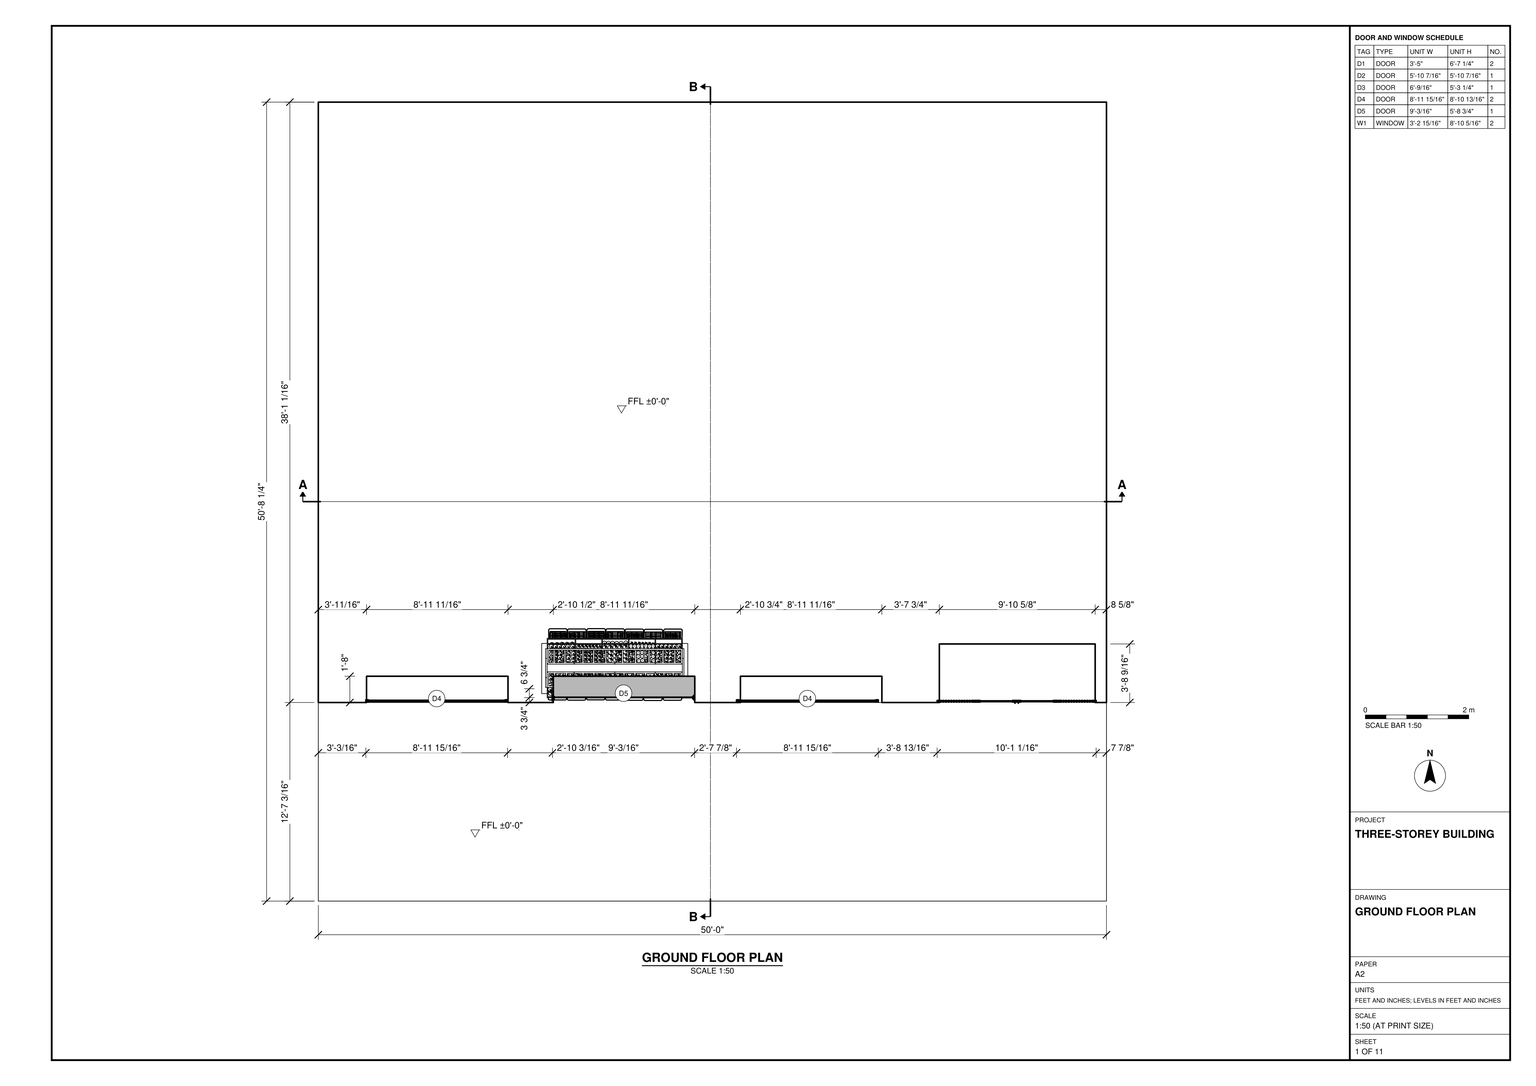
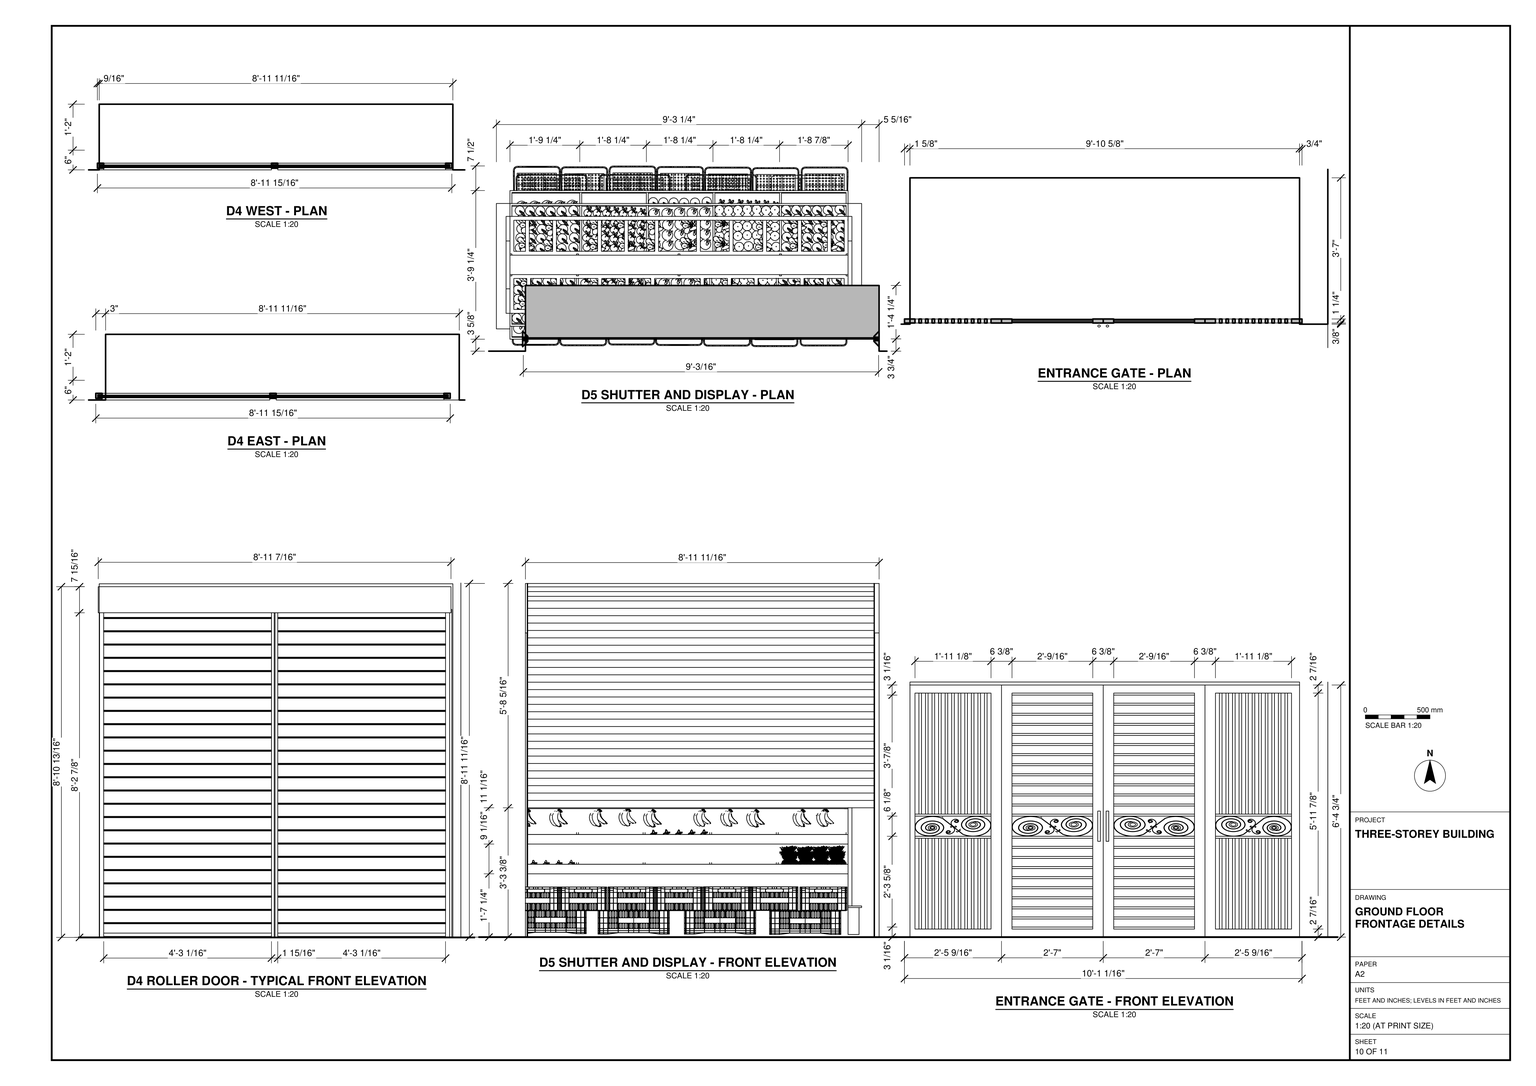
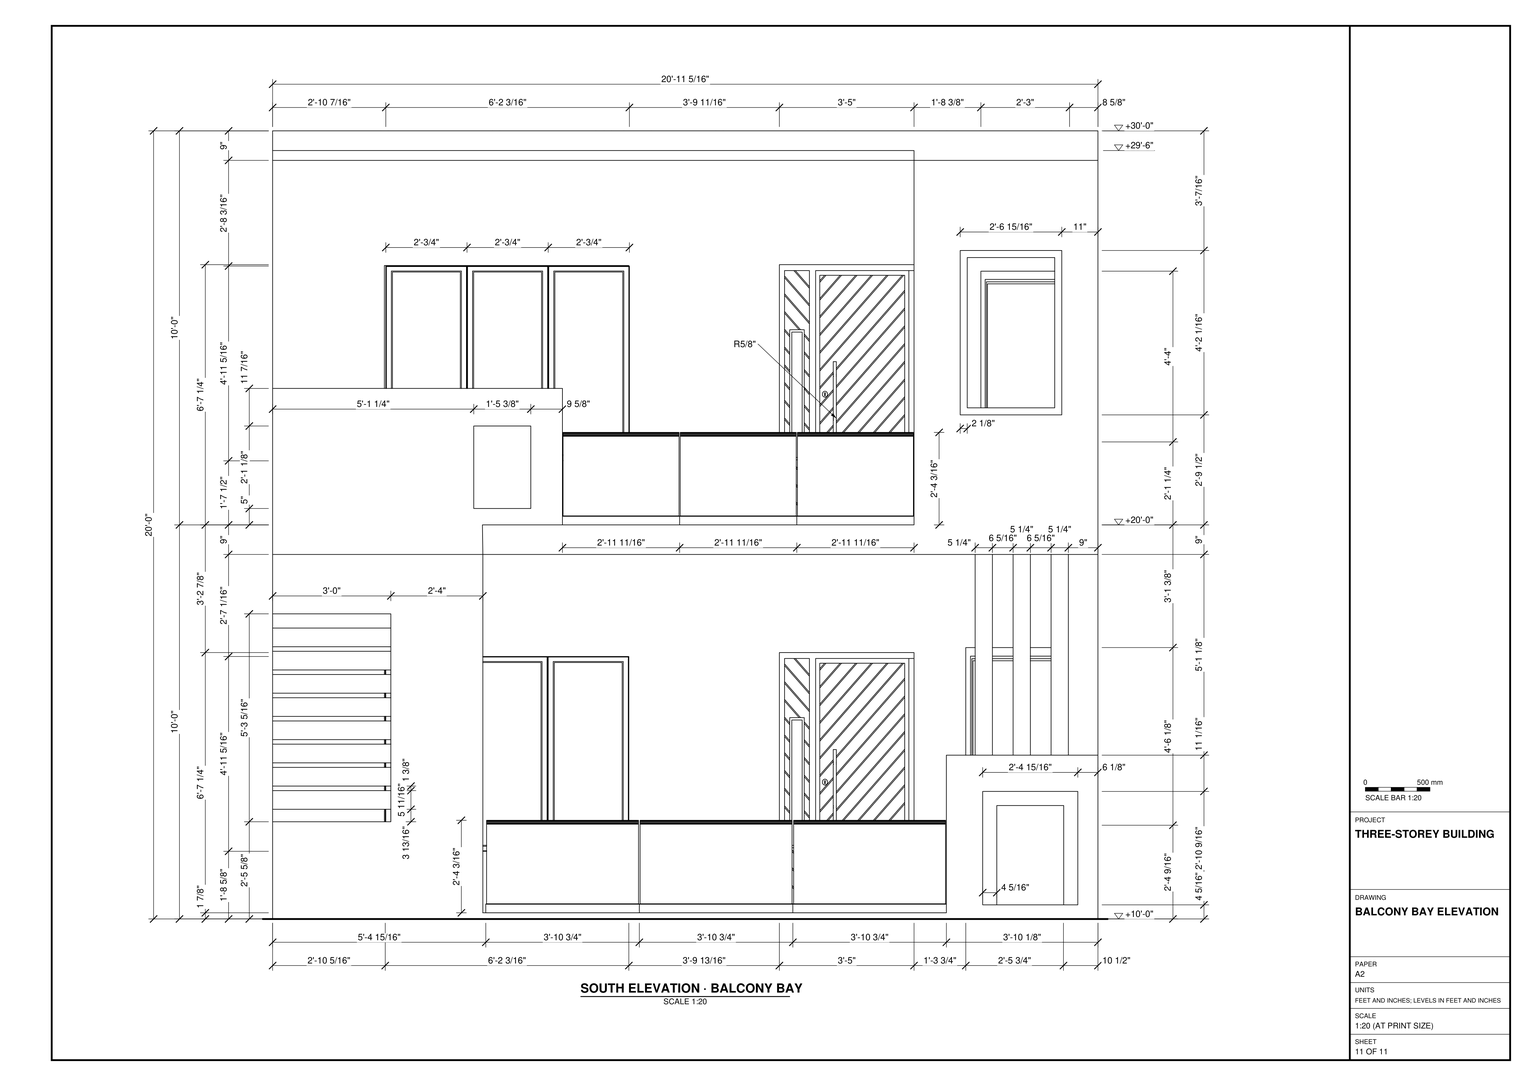
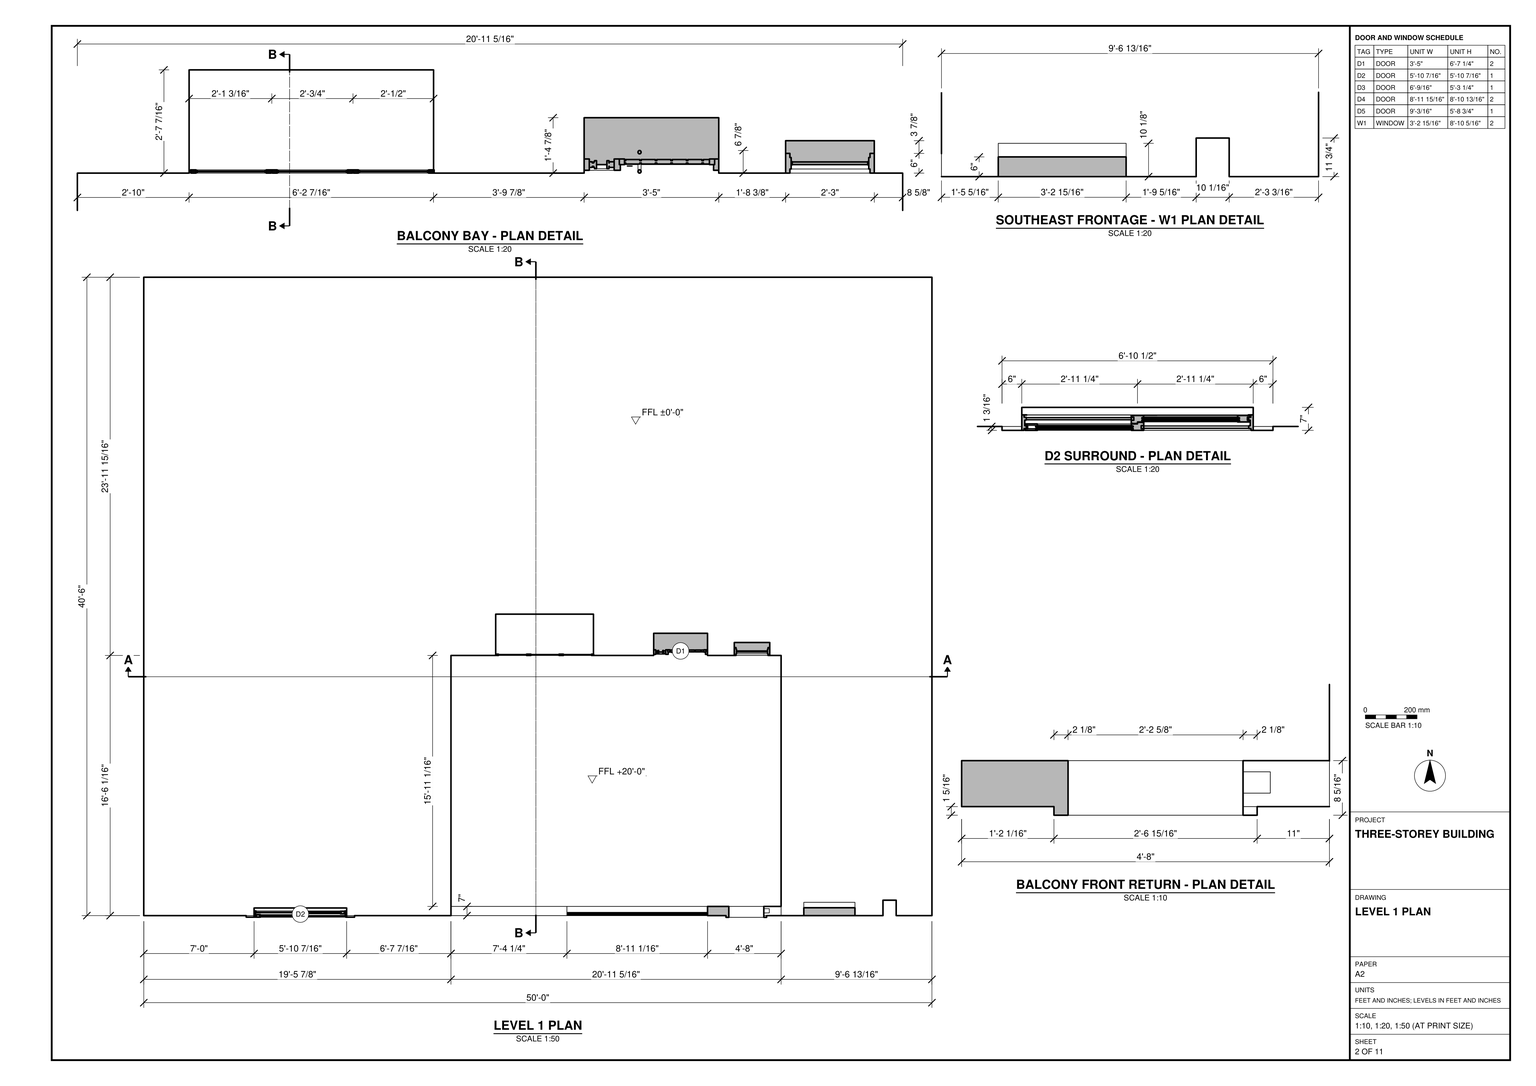
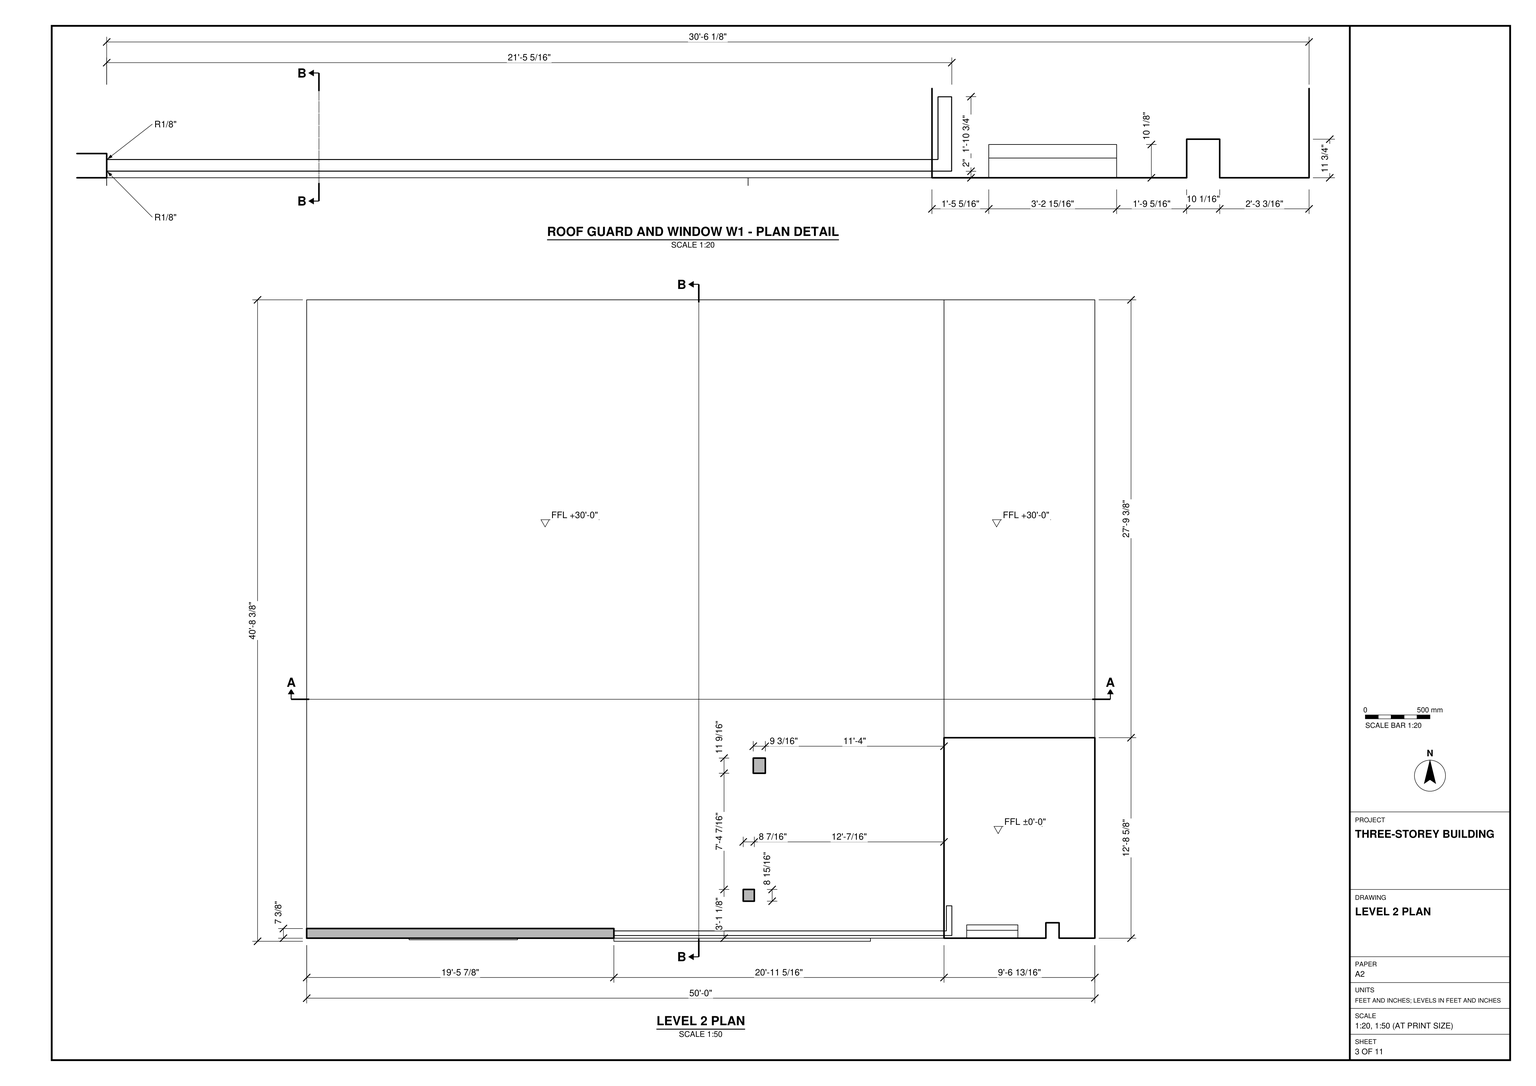
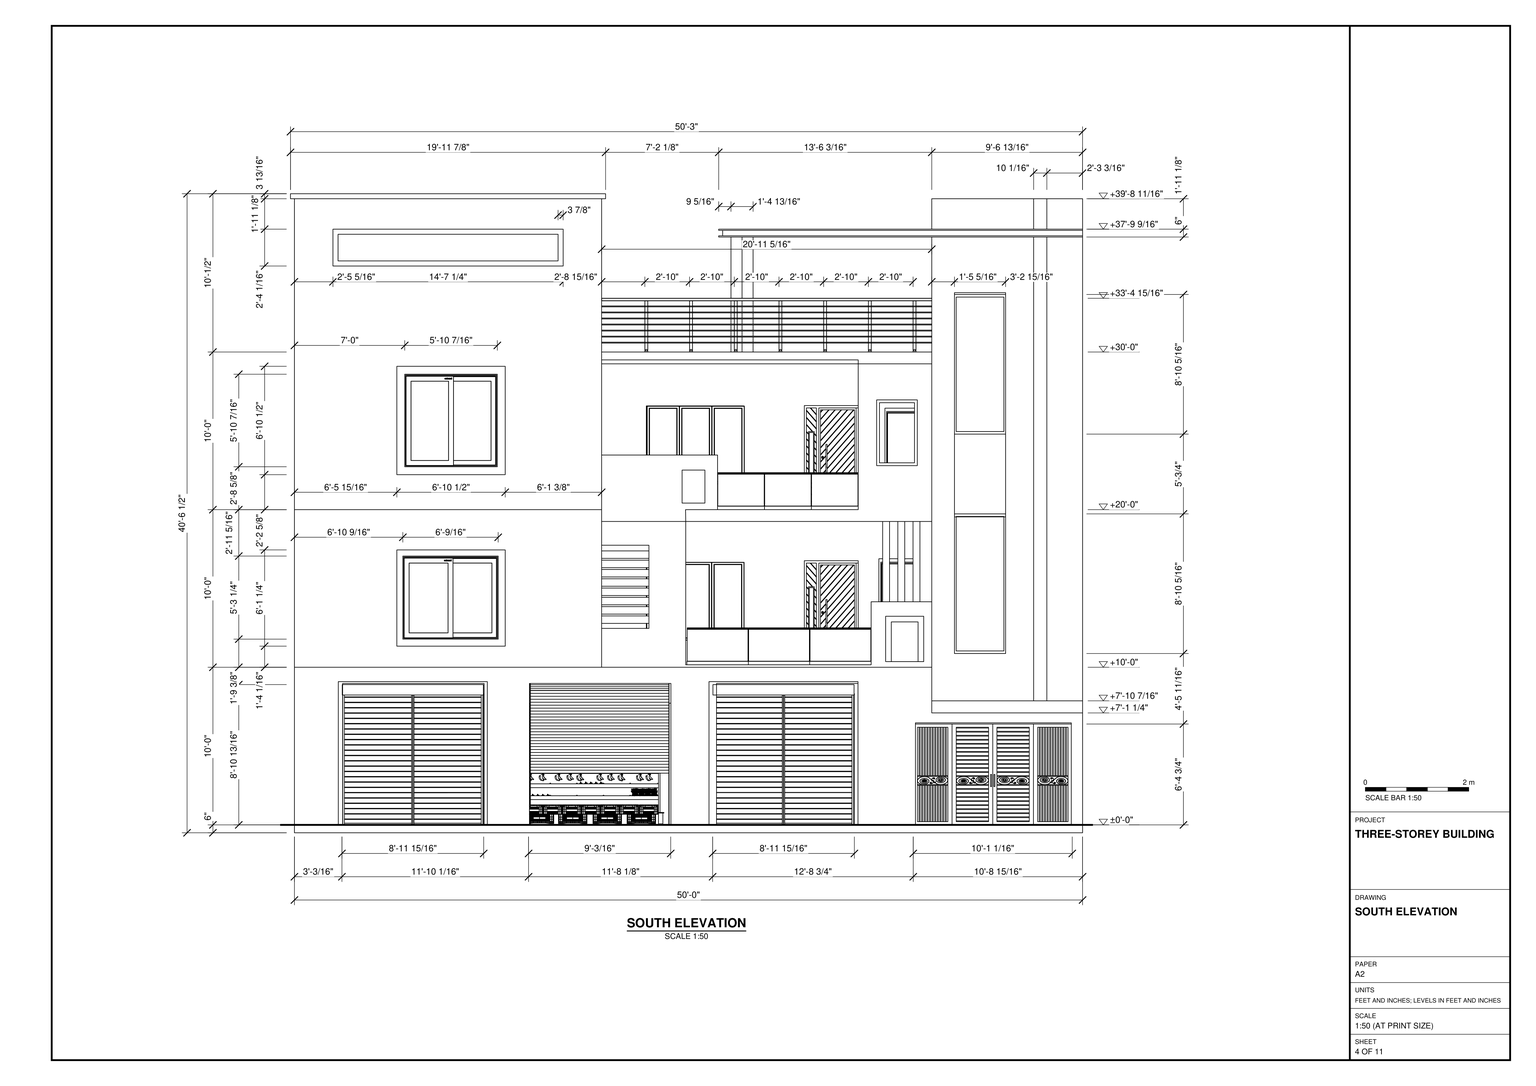
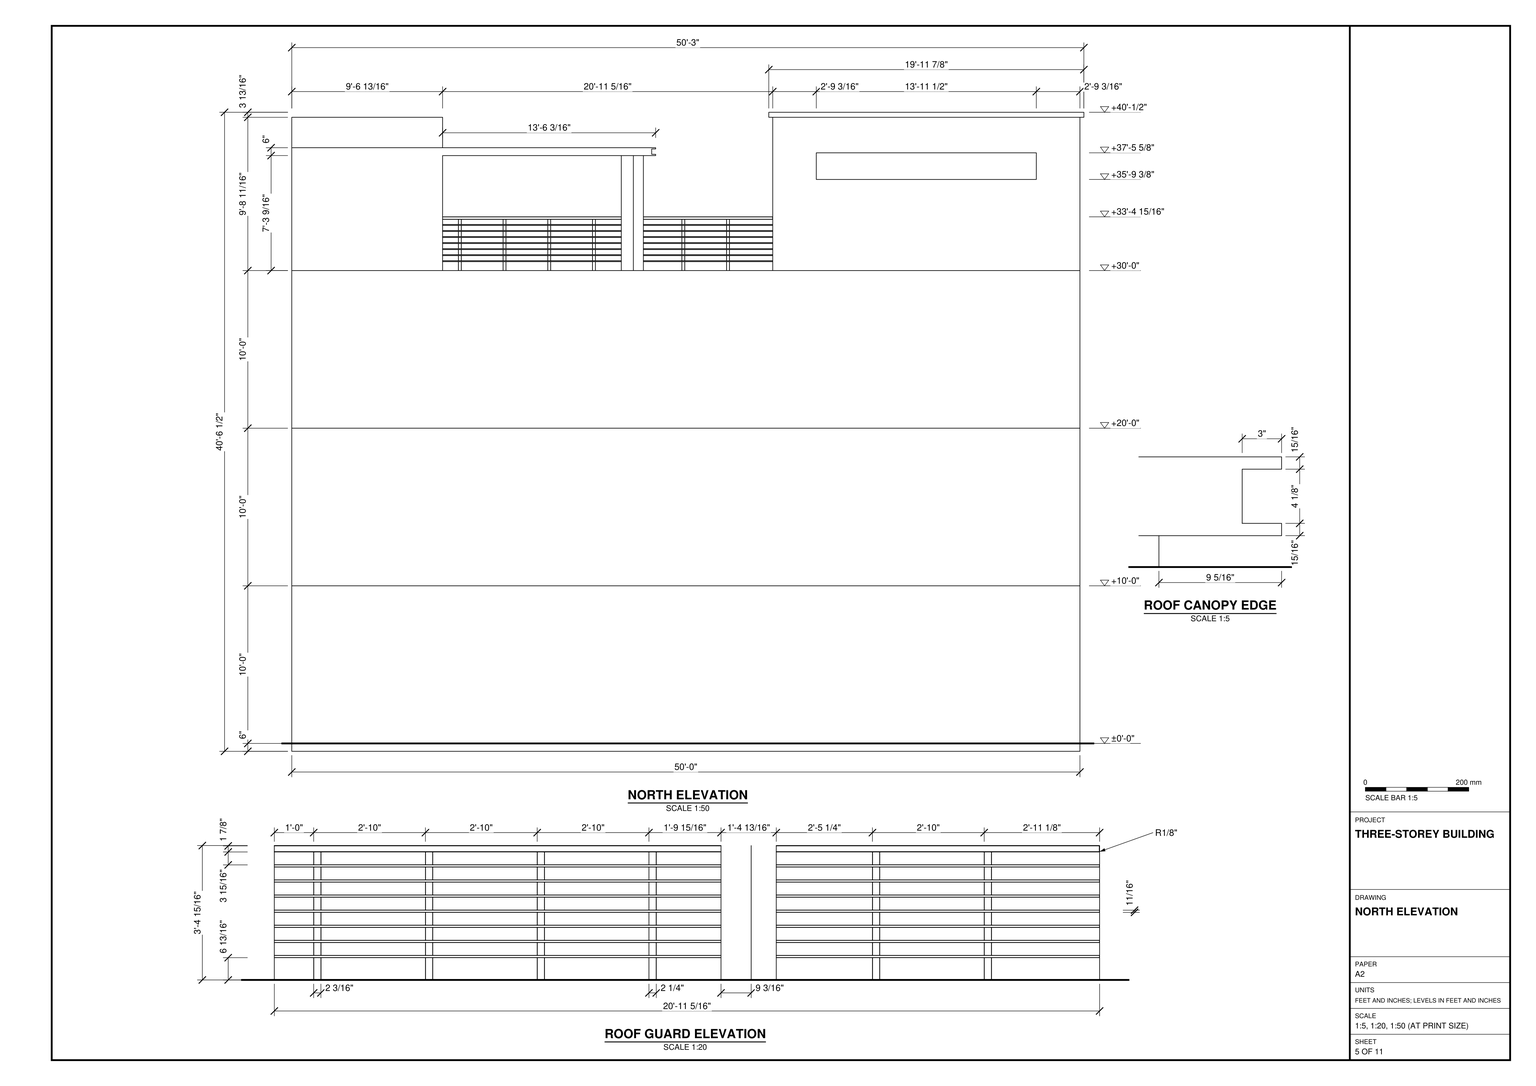
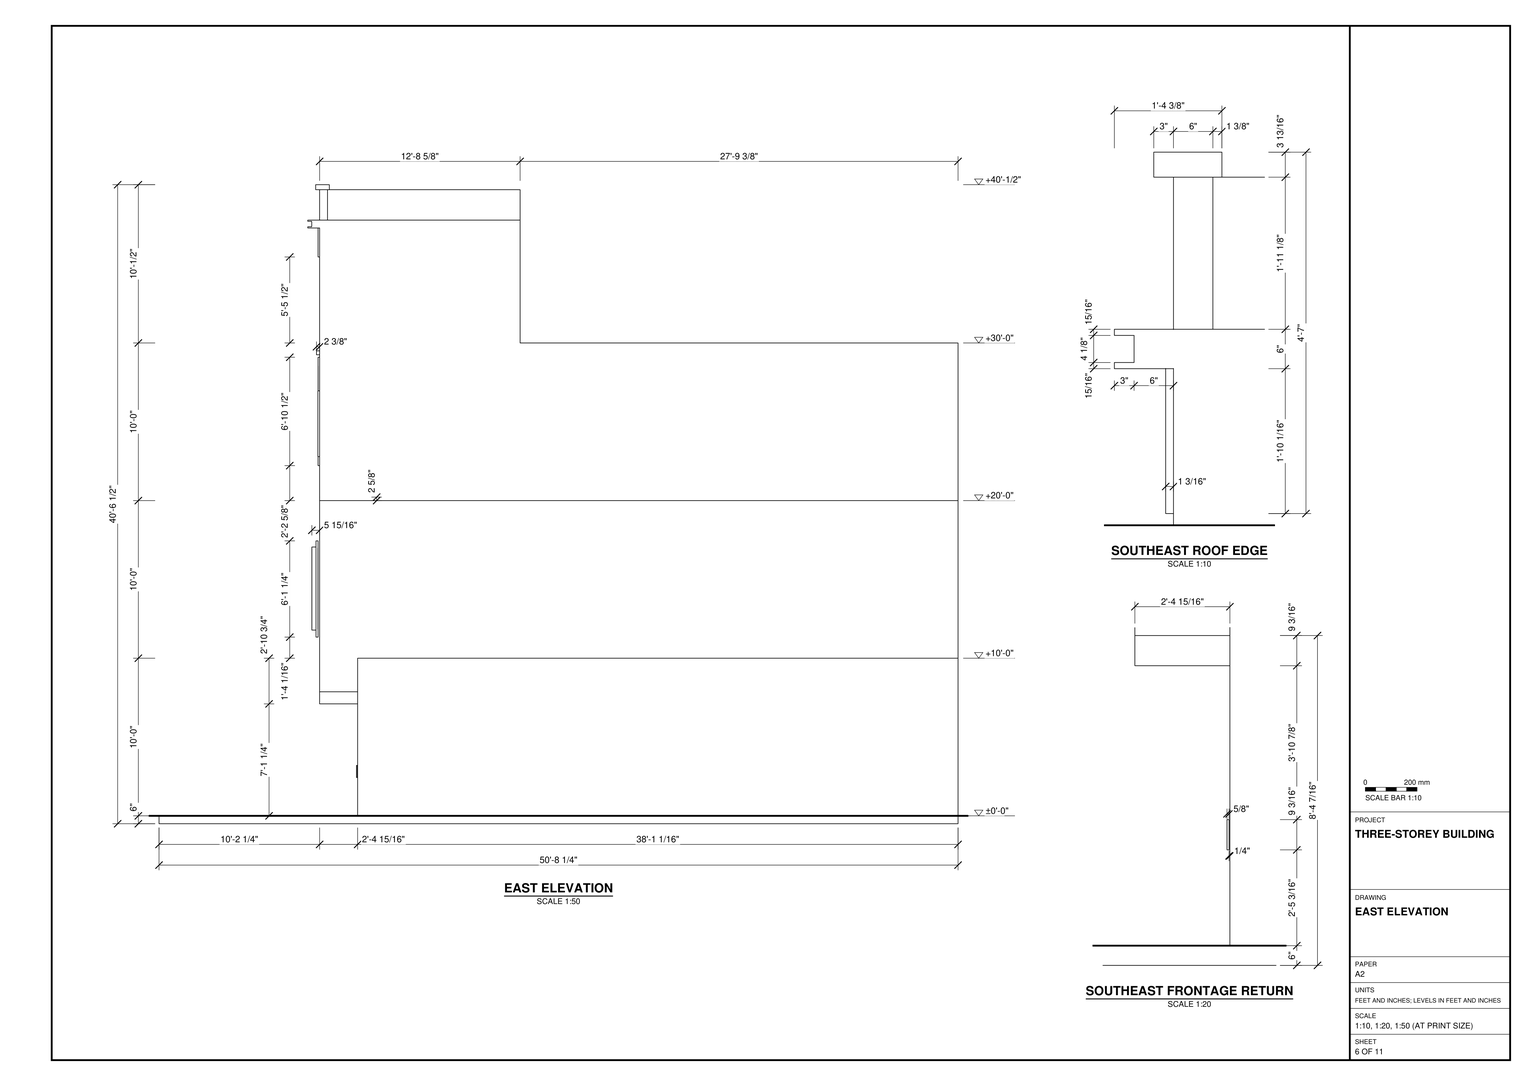
Build the three-storey building in SketchUp from task_files/diagram_01.pdf. Work in feet and inches. The overall model extents, including the area in front of the shops, are 50'-3" along X, 50'-8 1/4" along Y and 40'-6 1/2" along Z. Use the level references ±0'-0", +20'-0" and +30'-0" relative to the ground floor. Follow the plans and sections for wall thicknesses, floor slabs, roof profile and any stairs and landings.

Set the ground-floor frontage back from the south edge as drawn. From west to east, model a roller door, a shutter with a tiered shop display below it, a second roller door and the panelled entrance gate. Use the frontage details for the frames, slats and display joinery. Above, model the recessed balcony openings, doors, window units, solid wall returns and glass railings. Follow the balcony detail rather than duplicating the entire bay: the upper and lower railing spans differ. Include built-in joinery and main furniture where shown. Decor and loose items, including goods on the display, may be any suitable library components.

Keep shell elements such as walls, slabs and roof separate as groups or components. Group each furniture or joinery piece separately and use components for repeated parts. Save one SketchUp model as output_files/three_storey_building_with_shopfronts_and_balconies.skp.

# SketchUp Ruby script. Lengths in inches.
U = 1.inch
M = Sketchup.active_model
def pt(a) = Geom::Point3d.new(a.map { |v| v * U })
def face(e, loops, mat)
  f = e.add_face(loops[0].map { |a| pt(a) })
  loops[1..].each { |l| e.add_face(l.map { |a| pt(a) }).erase! }
  f.material = f.back_material = mat if mat
  f
end
# faces: each face lists its corners as indices into pts; further lists are holes
def faces(e, pts, list, mat = nil) = list.each { |f| face(e, (f[0].is_a?(Array) ? f : [f]).map { |l| l.map { |i| pts[i] } }, mat) }
# xy, xz, yz: faces in a plane at the given z, y or x. An outline is a flat list of corners, or four numbers for a rectangle; further outlines are holes
def ring(l) = l.size == 4 ? [[l[0], l[1]], [l[2], l[1]], [l[2], l[3]], [l[0], l[3]]] : l.each_slice(2).to_a
def flat(e, list, mat, &to3) = list.each { |f| face(e, (f[0].is_a?(Array) ? f : [f]).map { |l| ring(l).map { |u, v| to3.(u, v) } }, mat) }
def xy(e, z, list, mat = nil) = flat(e, list, mat) { |x, y| [x, y, z] }
def xz(e, y, list, mat = nil) = flat(e, list, mat) { |x, z| [x, y, z] }
def yz(e, x, list, mat = nil) = flat(e, list, mat) { |y, z| [x, y, z] }
def lines(e, pts, list) = list.each { |a, b| e.add_line(pt(pts[a]), pt(pts[b])) }
# prism: a flat outline (further loops are holes) pulled along v
def prism(e, loops, v, mat = nil)
  f = face(e, loops, mat); d = Geom::Vector3d.new(v.map { |x| x * U })
  f.pushpull(f.normal.samedirection?(d) ? d.length : -d.length)
end
def box(e, o, s, mat = nil) = prism(e, [[o, [o[0] + s[0], o[1], o[2]], [o[0] + s[0], o[1] + s[1], o[2]], [o[0], o[1] + s[1], o[2]]]], [0, 0, s[2]], mat)
def at(x, y, z, deg = 0) = Geom::Transformation.translation(pt([x, y, z])) * Geom::Transformation.rotation(ORIGIN, Z_AXIS, deg.degrees)
def axes(o, x, y, z) = Geom::Transformation.new([*x, 0, *y, 0, *z, 0, *pt(o).to_a, 1])
def part(name) = M.definitions.add(name)
# library, detail: a bought-in or finely detailed component or shape, given as its bounding box
def library(name, o, s) = part(name).tap { |d| box(d.entities, o, s) }
def detail(e, o, s) = box(e.add_group.entities, o, s)
def put(e, d, t, mat = nil) = e.add_instance(d, t).tap { |i| i.material = mat if mat }
def group(e, t, mat = nil) = e.add_group.tap { |g| g.transformation = t; g.material = mat if mat }.entities
root = M.entities
M.materials.add("GATE RAILINGS").color = [40, 40, 40]
M.materials.add("[0043_SaddleBrown]").color = [139, 69, 19]
M.materials.add("[0104_MediumBlue]").color = [0, 0, 205]
M.materials.add("[0135_DarkGray]").color = [81, 81, 81]
M.materials.add("[Color C04]").color = [255, 153, 50]
M.materials.add("[Color C08]").color = [102, 51, 0]
M.materials.add("[Color F03]").color = [178, 255, 101]
M.materials.add("[Color I05]").color = [0, 0, 255]
M.materials.add("[Color I08]").color = [0, 0, 102]
M.materials.add("[Color M07]").color = [58, 58, 58]
M.materials.add("[Concrete Pavers Block Multi]").color = [122, 137, 142]
M.materials.add("[Translucent Glass Gray]3").color = [128, 128, 128]
M.materials["[Translucent Glass Gray]3"].alpha = 0.3
M.materials.add("[Wood Cherry Original]").color = [152, 86, 42]
M.materials.add("[Wood Veneer 01]").color = [120, 70, 37]
c1 = library("Horizontal railing bar",[-171.26,0.98,-0.71],[237.2,23.72,0.71])
c2 = library("Railing post",[0,-1.77,-6.85],[2.07,1.28,39.37])
c3 = library("Group\#54",[-171.26,0,0],[238.19,24.7,1.97])
c4 = part("Balcony railing")
put(c4.entities,c1,at(44.24,-0.6875,35.43),"GATE RAILINGS")
put(c4.entities,c1,at(44.24,-0.6875,30.79),"GATE RAILINGS")
put(c4.entities,c1,at(44.24,-0.6875,26.14),"GATE RAILINGS")
put(c4.entities,c1,at(44.24,-0.6875,21.5),"GATE RAILINGS")
put(c4.entities,c1,at(44.24,-0.6875,16.85),"GATE RAILINGS")
put(c4.entities,c1,at(44.24,-0.6875,12.2),"GATE RAILINGS")
put(c4.entities,c1,at(44.24,-0.6875,7.56),"GATE RAILINGS")
put(c4.entities,c2,at(60.92,1.38,6.85))
put(c4.entities,c2,at(92.41,1.38,6.85))
put(c4.entities,c2,at(29.42,1.38,6.85))
put(c4.entities,c2,at(-2.07,1.38,6.85))
put(c4.entities,c2,at(-33.57,1.38,6.85))
put(c4.entities,c2,at(-65.07,1.38,6.85))
put(c4.entities,c2,at(-96.5625,1.38,6.85))
put(c4.entities,c3,at(44.24,-0.6875,39.37),"GATE RAILINGS")
c5 = library("Glass Railings(black Handrails)",[-57.04,-132.55,0],[169.29,2.52,28.17])
c6 = library("Door 7",[39.1,8.76,0],[51.18,7.87,86.61])
c7 = library("Glazed screen",[0,0,0],[135.86,2.83,115.35])
c8 = library("window3",[0,0,-0.05],[6,48,48.05])
c9 = library("AS-120-mm",[0,0,0],[70.47,4.72,70.47])
c10 = library("AS-120-mm\#1",[0,0,0],[72.58,4.72,63.25])
c11 = part("WINDOW")
xy(c11.entities,0,[[0,0,59.06,1.97]],"[Color M07]")
xy(c11.entities,1.97,[[1.97,0,57.09,0.98],[1.97,0.98,57.09,1.97]],"[Color M07]")
xy(c11.entities,104.33,[[1.97,0,57.09,0.98],[1.97,0.98,57.09,1.97]],"[Color M07]")
xy(c11.entities,106.3,[[0,0,59.06,1.97]],"[Color M07]")
xz(c11.entities,0,[[[0,0,59.06,106.3],[1.97,1.97,57.09,104.33]]],"[Color M07]")
xz(c11.entities,0.98,[[1.97,1.97,57.09,104.33]],"[Translucent Glass Gray]3")
xz(c11.entities,1.97,[[[0,0,59.06,106.3],[1.97,1.97,57.09,104.33]]],"[Color M07]")
yz(c11.entities,0,[[0,0,1.97,106.3]],"[Color M07]")
yz(c11.entities,1.97,[[0,1.97,0.98,104.33],[0.98,1.97,1.97,104.33]],"[Color M07]")
yz(c11.entities,57.09,[[0,1.97,0.98,104.33],[0.98,1.97,1.97,104.33]],"[Color M07]")
yz(c11.entities,59.06,[[0,0,1.97,106.3]],"[Color M07]")
c12 = library("Shop Roller Door",[0,0,0],[136,6,108])
c13 = library("Roller shop doors (shop 1)",[0,0,0],[119.37,22.8,123.23])
c14 = library("CONG+SAT",[0,-1.57,0],[119.37,3.14,98.43])
c15 = library("Group\#94",[0,0,0],[111.22,55.03,66.54])
xy(root,-2.52,[[3,0,603,608.25]])
xy(root,3.48,[[3,0,603,0,603,151.1875,594.39,151.1875,594.39,195.75,475.76,195.75,475.76,151.1875,432.03,151.1875,432.03,171.1875,324.34,171.1875,324.34,151.1875,289.59,151.1875,289.59,171.1875,181.9,171.1875,181.9,151.1875,147.4,151.1875,147.4,171.1875,39.71,171.1875,39.71,151.1875,3,151.1875],[3,151.1875,39.71,151.1875,39.71,171.1875,147.4,171.1875,147.4,151.1875,181.9,151.1875,181.9,171.1875,289.59,171.1875,289.59,151.1875,324.34,151.1875,324.34,171.1875,432.03,171.1875,432.03,151.1875,475.76,151.1875,475.76,195.75,594.39,195.75,594.39,151.1875,603,151.1875,603,608.25,3,608.25]])
xy(root,81.16,[[475.76,151.1875,594.39,195.75]])
xy(root,88.73,[[488.18,122.25,603,151.1875]],"[Color I05]")
xy(root,97.91,[[488.18,122.25,565.73,122.25,565.73,134,575.78,134,575.78,122.25,603,122.25,603,151.1875,488.18,151.1875],[565.73,122.25,575.78,134]])
xy(root,111.16,[[39.71,151.1875,147.4,171.1875],[181.9,151.1875,289.59,171.1875],[324.34,151.1875,432.03,171.1875]])
xy(root,123.48,[[3,122.25,3,151.1875,488.18,151.1875,488.18,122.75,236.87,122.75,236.87,122.25],[3,151.1875,3,608.25,603,608.25,603,151.1875,488.18,151.1875,488.18,320.3125,236.87,320.3125,236.87,151.1875]])
xy(root,125.35,[[300.88,122.75,442.03,130.25],[236.87,130.25,488.18,320.3125],[391.18,320.3125,432.18,349.375]])
xy(root,127.77,[[453.09,122.75,457.38,125.1875],[477.75,122.75,482.05,125.1875]])
xy(root,133.95,[[505.47,122.25,544.4,128.25]])
xy(root,139.54,[[80.96,119.5,163.46,121.0625]])
xy(root,144.08,[[270.9,320.3125,345.34,351.3125]])
xy(root,144.88,[[86.3125,119.5,158.12,121.0625]])
xy(root,152.0625,[[447.94,320.3125,477.69,331.125]])
xy(root,153.08,[[236.87,122.75,272.87,130.25]],"[0135_DarkGray]")
xy(root,156.875,[[236.87,123.49,275.24,127.68]])
xy(root,158.02,[[457.38,122.75,477.75,125.1875]])
xy(root,162.3125,[[453.09,122.75,482.05,125.1875]])
xy(root,162.5625,[[236.87,123.49,275.24,127.68]],"[0135_DarkGray]")
xy(root,163.95,[[236.87,123.49,275.68,127.68]])
xy(root,169.63,[[236.87,123.49,275.68,127.68]],"[0135_DarkGray]")
xy(root,171.02,[[236.87,123.49,277.43,127.68]])
xy(root,173.35,[[[442.03,122.75,488.18,130.25],[450.79,124.3,456.05,127.55],[462.35,124.3,467.61,127.55],[473.91,124.3,479.17,127.55]]])
xy(root,176.7,[[236.87,123.49,277.43,127.68]],"[0135_DarkGray]")
xy(root,178.09,[[236.87,123.49,275.81,127.68]])
xy(root,183.78,[[236.87,123.49,275.81,127.68]],"[0135_DarkGray]")
xy(root,185.16,[[236.87,123.49,274.62,127.68]])
xy(root,190.85,[[236.87,123.49,274.62,127.68]],"[0135_DarkGray]")
xy(root,192.23,[[236.87,123.49,274.37,127.68]])
xy(root,197.92,[[236.87,123.49,274.37,127.68]],"[0135_DarkGray]")
xy(root,199.3,[[236.87,123.49,272.87,127.68]])
xy(root,203.4,[[270.9,320.3125,345.34,351.3125]])
xy(root,204.6,[[391.18,320.3125,432.18,349.375]])
xy(root,204.99,[[236.87,123.49,272.87,127.68]],"[0135_DarkGray]")
xy(root,206.125,[[447.94,320.3125,477.69,331.125]])
xy(root,206.375,[[236.87,123.49,272.87,127.68]])
xy(root,207.46,[[86.3125,119.5,158.12,121.0625]])
xy(root,212.0625,[[236.87,123.49,272.87,127.68]],"[0135_DarkGray]")
xy(root,212.81,[[80.96,119.5,163.46,121.0625]])
xy(root,216.39,[[236.87,122.75,272.87,130.25]])
xy(root,234.48,[[236.87,122.25,300.88,122.75],[300.88,122.25,300.88,130.25,236.87,130.25,236.87,320.3125,488.18,320.3125,488.18,122.25]])
xy(root,235.66,[[462.35,124.3,467.61,127.55]])
xy(root,235.73,[[450.79,124.3,456.05,127.55]])
xy(root,236.1,[[473.91,124.3,479.17,127.55]])
xy(root,237.97,[[505.47,122.25,544.4,128.25]])
xy(root,243.48,[[325.12,122.25,432.18,129.25],[236.87,129.25,488.18,129.25,488.18,320.3125,432.18,320.3125,432.18,337.1875,391.18,337.1875,391.18,320.3125,236.87,320.3125]])
xy(root,248.47,[[298.11,122.25,315.49,123.875]])
xy(root,263.15,[[270.9,320.3125,345.34,351.75]])
xy(root,268.74,[[452.54,320.3125,479.54,330.1875]])
xy(root,270.1,[[80.96,121.0625,163.46,122.25]])
xy(root,273.59,[[298.11,122.25,315.49,123.875]])
xy(root,276.12,[[86.98,121.0625,157.45,128.0625]])
xy(root,276.98,[[446.23,120.9375,477.17,122.25]])
xy(root,279.125,[[448.38,120.9375,475.02,129.25]])
xy(root,285.04,[[236.87,122.25,325.12,129.25]])
xy(root,300.97,[[505.47,122.25,544.4,128.25]])
xy(root,320.74,[[452.54,320.3125,479.54,330.1875]])
xy(root,322.46,[[270.9,320.3125,345.34,351.75]])
xy(root,322.73,[[391.18,320.3125,432.18,337.1875]])
xy(root,324.89,[[448.38,120.9375,475.02,129.25]])
xy(root,327.04,[[446.23,120.9375,477.17,122.25]])
xy(root,346.58,[[86.98,121.0625,157.45,128.0625]])
xy(root,352.6,[[80.96,121.0625,163.46,122.25]])
xy(root,354.48,[[236.87,119.875,236.87,320.3125,488.18,320.3125,488.18,129.25,432.18,129.25,432.18,119.875]])
xy(root,357.48,[[236.87,119.875,432.18,122.25]])
xy(root,363.48,[[[236.87,122.25,488.18,122.25,488.18,608.25,3,608.25,3,129.625,236.87,129.625],[342.97,247.82,352.16,259.36],[335.33,150.42,343.76,159.36]],[488.18,274.875,603,608.25]])
xy(root,408.64,[[505.47,122.25,544.4,128.25]])
xy(root,428.95,[[32.33,121.0625,207.58,122.25]])
xy(root,432.83,[[36.22,121.0625,203.7,129.625]])
xy(root,451.01,[[335.33,150.42,343.76,159.36]])
xy(root,451.01,[[[325.99,113.25,325.99,274.875,488.18,274.875,488.18,122.25,565.73,122.25,565.73,134,575.78,134,575.78,122.25,603,122.25,603,113.25],[362.8125,153.49,456.0625,226.68],[342.97,247.82,352.16,259.36],[335.33,150.42,343.76,159.36]]],"[Color M07]")
xy(root,451.95,[[325.99,113.25,603,113.25,603,116.25,328.99,116.25,328.99,274.875,325.99,274.875]],"[Color M07]")
xy(root,453.13,[[36.22,121.0625,203.7,129.625]])
xy(root,456.07,[[325.99,113.25,325.99,274.875,328.99,274.875,328.99,116.25,603,116.25,603,113.25]],"[Color M07]")
xy(root,457.01,[[[325.99,113.25,603,113.25,603,128.25,575.78,128.25,575.78,134,565.73,134,565.73,128.25,488.18,128.25,488.18,274.875,325.99,274.875],[362.8125,153.49,456.0625,226.68]],[32.33,121.0625,207.58,122.25],[488.18,128.25,488.18,274.875,603,274.875,603,128.25,575.78,128.25,575.78,134,565.73,134,565.73,128.25]])
xy(root,480.16,[[0,119.25,239.87,122.25],[0,122.25,3,129.625],[3,122.25,236.87,129.625],[236.87,122.25,239.87,129.625]])
xy(root,480.16,[[488.18,128.25,565.73,128.25,565.73,134,575.78,134,575.78,128.25,603,128.25,603,274.875,488.18,274.875]],"[Concrete Pavers Block Multi]")
xy(root,483.98,[[0,119.25,239.87,129.625]])
xz(root,0,[[3,-2.52,603,3.48]])
xz(root,113.25,[[325.99,451.01,603,451.95],[325.99,456.07,603,457.01]])
xz(root,116.25,[[328.99,451.95,603,456.07]],"[Color C08]")
xz(root,119.25,[[0,480.16,239.87,483.98]])
xz(root,119.5,[[[80.96,139.54,163.46,212.81],[86.3125,144.88,158.12,207.46]]])
xz(root,119.875,[[236.87,354.48,432.18,357.48]])
xz(root,120.9375,[[[446.23,276.98,477.17,327.04],[448.38,279.125,475.02,324.89]]])
xz(root,121.0625,[[[80.96,139.54,163.46,212.81],[86.3125,144.88,158.12,207.46]],[86.3125,144.88,158.12,207.46],[[80.96,270.1,163.46,352.6],[86.98,276.12,157.45,346.58]],[[32.33,428.95,207.58,457.01],[36.22,432.83,203.7,453.13]]])
xz(root,122.25,[[[236.87,234.48,300.88,234.48,300.75,243.48,325.12,243.48,325.12,285.04,236.87,285.04],[298.11,248.47,315.49,273.59]]])
xz(root,122.25,[[[300.88,234.48,488.18,234.48,488.18,354.48,432.18,354.48,432.18,243.48,300.75,243.48],[446.23,276.98,477.17,327.04]],[432.18,354.48,488.18,354.48,488.18,363.48,236.87,363.48,236.87,357.48,432.18,357.48]],"[Color F03]")
xz(root,122.25,[[488.18,88.73,603,97.91]],"[Color I05]")
xz(root,122.25,[[3,123.48,236.87,243.48],[505.47,237.97,544.4,300.97]],"[Color I08]")
xz(root,122.25,[[[488.18,97.91,565.73,451.01],[505.47,133.95,544.4,408.64]],[575.78,97.91,603,451.01],[[3,243.48,236.87,480.16],[80.96,270.1,163.46,352.6],[32.33,428.95,207.58,457.01]]],"[Concrete Pavers Block Multi]")
xz(root,122.75,[[[236.87,123.48,488.18,123.48,488.18,173.35,442.03,173.35,442.03,125.35,300.88,125.35,300.88,234.48,236.87,234.48,236.87,216.39,272.87,216.39,272.87,153.08,236.87,153.08],[453.09,127.77,482.05,162.3125]],[457.38,127.77,477.75,158.02]])
xz(root,123.49,[[236.87,156.875,275.24,162.5625],[236.87,163.95,275.68,169.63],[236.87,171.02,277.43,176.7],[236.87,178.09,275.81,183.78],[236.87,185.16,274.62,190.85],
  [236.87,192.23,274.37,197.92],[236.87,199.3,272.87,204.99],[236.87,206.375,272.87,212.0625]],"[0135_DarkGray]")
xz(root,123.875,[[298.11,248.47,315.49,273.59]],"[0104_MediumBlue]")
xz(root,124.3,[[450.79,173.35,456.05,235.73],[462.35,173.35,467.61,235.66],[473.91,173.35,479.17,236.1]],"[0043_SaddleBrown]")
xz(root,125.1875,[[453.09,127.77,457.38,127.77,457.38,158.02,477.75,158.02,477.75,127.77,482.05,127.77,482.05,162.3125,453.09,162.3125]],"[0104_MediumBlue]")
xz(root,127.55,[[450.79,173.35,456.05,235.73],[462.35,173.35,467.61,235.66],[473.91,173.35,479.17,236.1]],"[0043_SaddleBrown]")
xz(root,127.68,[[236.87,156.875,275.24,162.5625],[236.87,163.95,275.68,169.63],[236.87,171.02,277.43,176.7],[236.87,178.09,275.81,183.78],[236.87,185.16,274.62,190.85],
  [236.87,192.23,274.37,197.92],[236.87,199.3,272.87,204.99],[236.87,206.375,272.87,212.0625]],"[0135_DarkGray]")
xz(root,128.0625,[[86.98,276.12,157.45,346.58]])
xz(root,128.25,[[505.47,133.95,544.4,237.97],[505.47,237.97,544.4,300.97],[505.47,300.97,544.4,408.64]])
xz(root,128.25,[[488.18,457.01,565.73,480.16],[575.78,457.01,603,480.16]],"[Concrete Pavers Block Multi]")
xz(root,129.25,[[236.87,243.48,325.12,285.04],[[432.18,243.48,488.18,354.48],[448.38,279.125,475.02,324.89]]])
xz(root,129.625,[[[3,363.48,236.87,480.16],[36.22,432.83,203.7,453.13]],[0,480.16,239.87,483.98]])
xz(root,130.25,[[236.87,125.35,300.88,125.35,300.88,234.48,236.87,234.48,236.87,216.39,272.87,216.39,272.87,153.08,236.87,153.08],[442.03,125.35,488.18,173.35]])
xz(root,134,[[565.73,457.01,575.78,480.16]],"[Wood Cherry Original]")
xz(root,134,[[565.73,97.91,575.78,451.01]],"[Wood Veneer 01]")
xz(root,150.42,[[335.33,363.48,343.76,451.01]],"[Color C04]")
xz(root,151.1875,[[3,3.48,39.71,3.48,39.71,111.16,147.4,111.16,147.4,3.48,181.9,3.48,181.9,111.16,289.59,111.16,289.59,3.48,324.34,3.48,324.34,111.16,432.03,111.16,432.03,3.48,475.76,3.48,475.76,81.16,594.39,81.16,594.39,3.48,603,3.48,603,88.73,488.18,88.73,488.18,123.48,3,123.48],[488.18,88.73,603,97.91],[488.18,97.91,603,123.48]])
xz(root,153.49,[[362.8125,451.01,456.0625,457.01]],"[Color M07]")
xz(root,159.36,[[335.33,363.48,343.76,451.01]],"[Color C04]")
xz(root,171.1875,[[39.71,3.48,147.4,111.16],[181.9,3.48,289.59,111.16],[324.34,3.48,432.03,111.16]])
xz(root,195.75,[[475.76,3.48,594.39,81.16]])
xz(root,226.68,[[362.8125,451.01,456.0625,457.01]],"[Color M07]")
xz(root,247.82,[[342.97,363.48,352.16,451.01]],"[Color C04]")
xz(root,259.36,[[342.97,363.48,352.16,451.01]],"[Color C04]")
xz(root,274.875,[[488.18,363.48,488.18,451.01,325.99,451.01,325.99,451.95,328.99,451.95,328.99,456.07,325.99,456.07,325.99,457.01,603,457.01,603,363.48],[488.18,457.01,603,480.16]])
xz(root,320.3125,[[236.87,123.48,488.18,125.35]])
xz(root,320.3125,[[[236.87,125.35,391.18,125.35,391.18,204.6,432.18,204.6,432.18,125.35,488.18,125.35,488.18,234.48,236.87,234.48],[270.9,144.08,345.34,203.4],[447.94,152.0625,477.69,206.125]],[[236.87,243.48,391.18,243.48,391.18,322.73,432.18,322.73,432.18,243.48,488.18,243.48,488.18,354.48,236.87,354.48],[270.9,263.15,345.34,322.46],[452.54,268.74,479.54,320.74]]],"[Color F03]")
xz(root,330.1875,[[452.54,268.74,479.54,320.74]])
xz(root,331.125,[[447.94,152.0625,477.69,206.125]])
xz(root,337.1875,[[391.18,243.48,432.18,322.73]])
xz(root,349.375,[[391.18,125.35,432.18,204.6]])
xz(root,351.3125,[[270.9,144.08,345.34,203.4]])
xz(root,351.75,[[270.9,263.15,345.34,322.46]])
xz(root,608.25,[[3,-2.52,603,3.48],[3,3.48,603,123.48],[3,123.48,603,243.48],[3,243.48,603,363.48]])
yz(root,0,[[119.25,480.16,129.625,483.98]])
yz(root,3,[[0,-2.52,608.25,3.48],[151.1875,3.48,608.25,123.48],[122.25,123.48,608.25,243.48],[122.25,243.48,122.25,480.16,129.625,480.16,129.625,363.48,608.25,363.48,608.25,243.48]])
yz(root,32.33,[[121.0625,428.95,122.25,457.01]])
yz(root,36.22,[[121.0625,432.83,129.625,453.13]])
yz(root,39.71,[[151.1875,3.48,171.1875,111.16]])
yz(root,80.96,[[119.5,139.54,121.0625,212.81],[121.0625,270.1,122.25,352.6]])
yz(root,86.3125,[[119.5,144.88,121.0625,207.46]])
yz(root,86.98,[[121.0625,276.12,128.0625,346.58]])
yz(root,147.4,[[151.1875,3.48,171.1875,111.16]])
yz(root,157.45,[[121.0625,276.12,128.0625,346.58]])
yz(root,158.12,[[119.5,144.88,121.0625,207.46]])
yz(root,163.46,[[119.5,139.54,121.0625,212.81],[121.0625,270.1,122.25,352.6]])
yz(root,181.9,[[151.1875,3.48,171.1875,111.16]])
yz(root,203.7,[[121.0625,432.83,129.625,453.13]])
yz(root,207.58,[[121.0625,428.95,122.25,457.01]])
yz(root,236.87,[[122.25,123.48,122.75,153.08],[151.1875,123.48,320.3125,125.35],[130.25,125.35,320.3125,234.48],[122.25,216.39,122.75,234.48],[129.25,243.48,320.3125,243.48,320.3125,354.48,122.25,354.48,122.25,285.04,129.25,285.04],
  [119.875,354.48,122.25,357.48],[122.25,363.48,129.625,480.16]])
yz(root,236.87,[[[122.25,153.08,130.25,216.39],[123.49,206.375,127.68,212.0625],[123.49,199.3,127.68,204.99],[123.49,192.23,127.68,197.92],[123.49,185.16,127.68,190.85],[123.49,178.09,127.68,183.78],[123.49,171.02,127.68,176.7],[123.49,163.95,127.68,169.63],[123.49,156.875,127.68,162.5625]]],"[0135_DarkGray]")
yz(root,239.87,[[119.25,480.16,129.625,483.98]])
yz(root,270.9,[[320.3125,144.08,351.3125,203.4],[320.3125,263.15,351.75,322.46]])
yz(root,272.87,[[[122.75,153.08,130.25,216.39],[123.49,206.375,127.68,212.0625],[123.49,199.3,127.68,204.99]]])
yz(root,274.37,[[123.49,192.23,127.68,197.92]])
yz(root,274.62,[[123.49,185.16,127.68,190.85]])
yz(root,275.24,[[123.49,156.875,127.68,162.5625]])
yz(root,275.68,[[123.49,163.95,127.68,169.63]])
yz(root,275.81,[[123.49,178.09,127.68,183.78]])
yz(root,277.43,[[123.49,171.02,127.68,176.7]])
yz(root,289.59,[[151.1875,3.48,171.1875,111.16]])
yz(root,298.11,[[122.25,248.47,123.875,273.59]])
yz(root,300.88,[[122.75,125.35,130.25,234.48]])
yz(root,315.49,[[122.25,248.47,123.875,273.59]])
yz(root,324.34,[[151.1875,3.48,171.1875,111.16]])
yz(root,325.12,[[122.25,243.48,129.25,285.04]])
yz(root,325.99,[[113.25,451.01,274.875,451.95],[113.25,456.07,274.875,457.01]],"[Color M07]")
yz(root,328.99,[[116.25,451.95,274.875,456.07]],"[Color C08]")
yz(root,335.33,[[150.42,363.48,159.36,451.01]],"[Color C04]")
yz(root,342.97,[[247.82,363.48,259.36,451.01]],"[Color C04]")
yz(root,343.76,[[150.42,363.48,159.36,451.01]],"[Color C04]")
yz(root,345.34,[[320.3125,144.08,351.3125,203.4],[320.3125,263.15,351.75,322.46]])
yz(root,352.16,[[247.82,363.48,259.36,451.01]],"[Color C04]")
yz(root,362.8125,[[153.49,451.01,226.68,457.01]])
yz(root,391.18,[[320.3125,125.35,349.375,204.6],[320.3125,243.48,337.1875,322.73]])
yz(root,432.03,[[151.1875,3.48,171.1875,111.16]])
yz(root,432.18,[[320.3125,125.35,349.375,204.6],[122.25,243.48,129.25,354.48],[320.3125,243.48,337.1875,322.73],[119.875,354.48,122.25,357.48]])
yz(root,442.03,[[122.75,125.35,130.25,173.35]])
yz(root,446.23,[[120.9375,276.98,122.25,327.04]])
yz(root,447.94,[[320.3125,152.0625,331.125,206.125]])
yz(root,448.38,[[120.9375,279.125,129.25,324.89]])
yz(root,450.79,[[124.3,173.35,127.55,235.73]],"[0043_SaddleBrown]")
yz(root,452.54,[[320.3125,268.74,330.1875,320.74]])
yz(root,453.09,[[122.75,127.77,125.1875,162.3125]])
yz(root,456.05,[[124.3,173.35,127.55,235.73]],"[0043_SaddleBrown]")
yz(root,456.0625,[[153.49,451.01,226.68,457.01]],"[Color M07]")
yz(root,457.38,[[122.75,127.77,125.1875,158.02]])
yz(root,462.35,[[124.3,173.35,127.55,235.66]],"[0043_SaddleBrown]")
yz(root,467.61,[[124.3,173.35,127.55,235.66]],"[0043_SaddleBrown]")
yz(root,473.91,[[124.3,173.35,127.55,236.1]],"[0043_SaddleBrown]")
yz(root,475.02,[[120.9375,279.125,129.25,324.89]])
yz(root,475.76,[[151.1875,3.48,195.75,81.16]])
yz(root,477.17,[[120.9375,276.98,122.25,327.04]])
yz(root,477.69,[[320.3125,152.0625,331.125,206.125]])
yz(root,477.75,[[122.75,127.77,125.1875,158.02]])
yz(root,479.17,[[124.3,173.35,127.55,236.1]],"[0043_SaddleBrown]")
yz(root,479.54,[[320.3125,268.74,330.1875,320.74]])
yz(root,482.05,[[122.75,127.77,125.1875,162.3125]])
yz(root,488.18,[[122.25,97.91,151.1875,123.48],[122.25,123.48,122.75,125.35],[122.75,123.48,122.75,173.35,130.25,173.35,130.25,125.35,151.1875,125.35,151.1875,123.48],[151.1875,123.48,320.3125,125.35],[122.25,125.35,122.25,234.48,320.3125,234.48,320.3125,125.35,130.25,125.35,130.25,173.35,122.75,173.35,122.75,125.35],
  [129.25,243.48,320.3125,354.48],[122.25,363.48,274.875,451.01]])
yz(root,488.18,[[122.25,88.73,151.1875,97.91]],"[Color I05]")
yz(root,488.18,[[128.25,457.01,274.875,480.16]],"[Concrete Pavers Block Multi]")
yz(root,505.47,[[122.25,133.95,128.25,237.97],[122.25,237.97,128.25,300.97],[122.25,300.97,128.25,408.64]])
yz(root,544.4,[[122.25,133.95,128.25,237.97],[122.25,237.97,128.25,300.97],[122.25,300.97,128.25,408.64]])
yz(root,565.73,[[128.25,457.01,134,480.16]],"[Wood Cherry Original]")
yz(root,565.73,[[122.25,97.91,134,451.01]],"[Wood Veneer 01]")
yz(root,575.78,[[128.25,457.01,134,480.16]],"[Wood Cherry Original]")
yz(root,575.78,[[122.25,97.91,134,451.01]],"[Wood Veneer 01]")
yz(root,594.39,[[151.1875,3.48,195.75,81.16]])
yz(root,603,[[0,-2.52,608.25,3.48],[151.1875,3.48,608.25,123.48],[122.25,97.91,151.1875,97.91,151.1875,123.48,608.25,123.48,608.25,243.48,122.25,243.48],[122.25,243.48,608.25,243.48,608.25,363.48,274.875,363.48,274.875,457.01,113.25,457.01,113.25,456.07,116.25,456.07,116.25,451.95,113.25,451.95,113.25,451.01,122.25,451.01]])
yz(root,603,[[122.25,88.73,151.1875,97.91]],"[Color I05]")
yz(root,603,[[128.25,457.01,274.875,480.16]],"[Concrete Pavers Block Multi]")
put(root,c4,axes([374.1,124.86,363.48],[1.08039,0,0],[0,0.92,0],[0,0,0.99]))
put(root,c5,axes([361.2,254.8,243.48],[0.63239,0,0],[0,1,0],[0,0,1]))
put(root,c5,axes([349.04,255.3,125.35],[0.82843,0,0],[0,1,0],[0,0,1]))
put(root,c6,axes([359.86,312.65,125.35],[0.80108,0,0],[0,0.875,0],[0,0,0.91498]))
put(root,c6,axes([359.86,312.65,243.48],[0.80108,0,0],[0,0.875,0],[0,0,0.91498]))
put(root,c7,axes([271.16,320.3125,144.08],[0.546,0,0],[0,0.35,0],[0,0,0.51418]))
put(root,c7,axes([271.33,320.3125,262.99],[0.546,0,0],[0,0.35,0],[0,0,0.51418]))
put(root,c8,axes([477.69,320.3125,152.07],[0,1,0],[-0.61979,0,0],[0,0,1.12617]))
put(root,c8,axes([479.54,320.3125,268.8],[0,1,0],[-0.5625,0,0],[0,0,1.08221]))
put(root,c9,at(86.98,121.0625,276.12))
put(root,c10,at(85.54,116.34,144.88))
put(root,c11,axes([505.47,122.25,133.95],[0.65934,0,0],[0,5.15,0],[0,0,1]))
put(root,c11,axes([505.47,122.25,300.97],[0.65934,0,0],[0,5.15,0],[0,0,1]))
put(root,c12,axes([36.41,151.1875,3.48],[0.83403,0,0],[0,1,0],[0,0,1.01]))
put(root,c12,axes([318.6,151.1875,3.48],[0.83403,0,0],[0,1,0],[0,0,1.01]))
put(root,c13,axes([181,152.56,-2.52],[0.91,0,0],[0,0.94,0],[0,0,0.95258]))
put(root,c14,axes([474.09,151.53,3.48],[1.014,0,0],[0,0.78,0],[0,0,0.78]))
put(root,c15,axes([173.05,152.56,4.27],[1,0,0],[0,1,0],[0,0,0.61375]))
